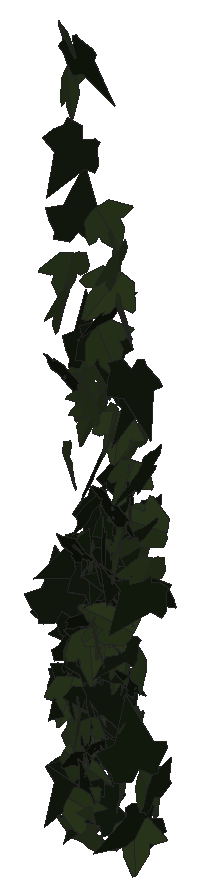
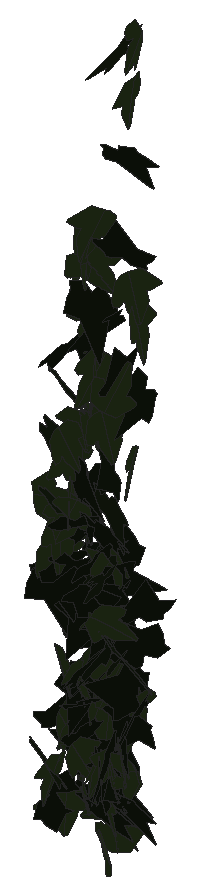
# SketchUp Ruby script. Lengths in inches.
U = 1.inch
M = Sketchup.active_model
def pt(a) = Geom::Point3d.new(a.map { |v| v * U })
def face(e, loops, mat)
  f = e.add_face(loops[0].map { |a| pt(a) })
  loops[1..].each { |l| e.add_face(l.map { |a| pt(a) }).erase! }
  f.material = f.back_material = mat if mat
  f
end
# faces: each face lists its corners as indices into pts; further lists are holes
def faces(e, pts, list, mat = nil) = list.each { |f| face(e, (f[0].is_a?(Array) ? f : [f]).map { |l| l.map { |i| pts[i] } }, mat) }
# xy, xz, yz: faces in a plane at the given z, y or x. An outline is a flat list of corners, or four numbers for a rectangle; further outlines are holes
def ring(l) = l.size == 4 ? [[l[0], l[1]], [l[2], l[1]], [l[2], l[3]], [l[0], l[3]]] : l.each_slice(2).to_a
def flat(e, list, mat, &to3) = list.each { |f| face(e, (f[0].is_a?(Array) ? f : [f]).map { |l| ring(l).map { |u, v| to3.(u, v) } }, mat) }
def xy(e, z, list, mat = nil) = flat(e, list, mat) { |x, y| [x, y, z] }
def xz(e, y, list, mat = nil) = flat(e, list, mat) { |x, z| [x, y, z] }
def yz(e, x, list, mat = nil) = flat(e, list, mat) { |y, z| [x, y, z] }
def lines(e, pts, list) = list.each { |a, b| e.add_line(pt(pts[a]), pt(pts[b])) }
# prism: a flat outline (further loops are holes) pulled along v
def prism(e, loops, v, mat = nil)
  f = face(e, loops, mat); d = Geom::Vector3d.new(v.map { |x| x * U })
  f.pushpull(f.normal.samedirection?(d) ? d.length : -d.length)
end
def box(e, o, s, mat = nil) = prism(e, [[o, [o[0] + s[0], o[1], o[2]], [o[0] + s[0], o[1] + s[1], o[2]], [o[0], o[1] + s[1], o[2]]]], [0, 0, s[2]], mat)
def at(x, y, z, deg = 0) = Geom::Transformation.translation(pt([x, y, z])) * Geom::Transformation.rotation(ORIGIN, Z_AXIS, deg.degrees)
def axes(o, x, y, z) = Geom::Transformation.new([*x, 0, *y, 0, *z, 0, *pt(o).to_a, 1])
def part(name) = M.definitions.add(name)
# library, detail: a bought-in or finely detailed component or shape, given as its bounding box
def library(name, o, s) = part(name).tap { |d| box(d.entities, o, s) }
def detail(e, o, s) = box(e.add_group.entities, o, s)
def put(e, d, t, mat = nil) = e.add_instance(d, t).tap { |i| i.material = mat if mat }
def group(e, t, mat = nil) = e.add_group.tap { |g| g.transformation = t; g.material = mat if mat }.entities
root = M.entities
M.materials.add("efeu1").color = [18, 25, 13]
M.materials.add("efeu2").color = [43, 57, 29]
c1 = part("ivyleaf_10")
p = [[0,0.5,-0.03],[-0.0625,2.02,-0.43],[-0.19,2.01,-0.46],[-0.54,1.05,-0.29],[-0.52,0.625,-0.18],[-0.83,0.76,-0.28],
  [-1.16,0.64,-0.33],[-1.15,0.33,-0.24],[-0.77,-0.39,0.02],[-0.3,-0.51,0.16],[0.04,-0.48,0.23],[-0.02,2.01,-0.4375],
  [-0.06,2.01,-0.43],[0.04,-0.49,0.23],[0.67,-0.49,0.14],[1.38,0.36,-0.2],[1.375,0.51,-0.24],[0.81,0.65,-0.19],
  [0.62,0.59,-0.15],[0.6,1.09,-0.28],[0.5,1.23,-0.31]]
faces(c1.entities,p,[[0,1,2,3,4,5,6,7,8,9,10],[11,12,0,13,14,15,16,17,18,19,20]],"efeu2")
c2 = part("ivyleaf_9")
p = [[1.54,2.16,1.25],[1.36,2.04,1.19],[-0.21,0.99,0.68],[-0.71,1.11,0.82],[-0.85,0.86,0.67],[-0.8,0.17,0.21],
  [-0.9,-0.01,0.1],[-0.67,-0.16,-0.02],[-0.08,-0.08,-0.05],[-0.03,-0.6,-0.4],[0.65,-0.88,-0.66],[0.83,-0.6,-0.49],
  [1.29,-0.42,-0.43],[1.8125,-0.07,-0.26],[1.21,0.44,0.15]]
faces(c2.entities,p,[[0,1,2,3,4,5,6,7,8,9,10,11,12,13,14]],"efeu1")
put(root,c1,axes([507.67,132.25,225.15],[-0.67169,0.30588,0.55125],[-0.57014,0.04902,-0.7219],[-0.26904,-0.86755,0.15357]))
put(root,c1,axes([506.41,132.4,240.61],[-0.63709,0.59964,-0.19778],[0.12594,-0.15195,-0.87449],[-0.66763,-0.60088,0.02377]))
put(root,c2,axes([506.32,132.27,215.31],[-0.63529,-0.37926,0.39302],[0.33878,0.21084,0.72786],[-0.46859,0.66662,-0.00661]))
put(root,c1,axes([507.2,132.45,210.73],[-0.86644,-0.09764,0.1844],[-0.173,-0.13686,-0.83213],[0.13365,-0.81014,0.11835]))
put(root,c1,axes([506.57,132.55,211.79],[0.53988,0.54531,-0.22704],[-0.16249,-0.15823,-0.76935],[-0.61321,0.52202,0.00397]))
put(root,c1,axes([507.625,132.41,214.31],[0.4981,0.73589,0.03065],[0.02054,0.02311,-0.8886],[-0.73624,0.49851,-0.00405]))
put(root,c1,axes([509.375,132.2,229.53],[-0.58306,0.57776,0.226],[-0.1394,0.17665,-0.82195],[-0.65192,-0.55451,-0.02637]))
put(root,c2,axes([507.05,133.03,207.83],[-0.06531,-0.25331,0.74015],[0.0799,-0.71251,-0.25721],[0.81193,0.04974,0.08485]))
put(root,c1,axes([508.6,132.67,230.33],[0.75093,0.29794,-0.48827],[-0.45735,-0.17118,-0.80784],[-0.34351,0.87921,0.00817]))
put(root,c1,axes([506.71,132.2,222.07],[-0.51143,0.56113,0.30999],[-0.22253,0.21604,-0.76342],[-0.64913,-0.51616,0.01748]))
put(root,c2,axes([506.87,132.48,240.15],[0.61355,-0.6211,-0.17687],[-0.01821,0.21235,-0.86517],[0.69524,0.55368,0.13342]))
put(root,c1,axes([508.78,132.77,218.96],[0.59224,-0.52273,0.26011],[0.21093,-0.15748,-0.78764],[0.58923,0.58177,0.02051]))
put(root,c1,axes([508.43,132.19,228.03],[0.27209,0.82406,0.33922],[-0.05181,0.3687,-0.85414],[-0.88964,0.23056,0.15349]))
put(root,c1,axes([508.94,132.8125,215.17],[0.25706,0.28657,0.81958],[-0.66136,-0.48916,0.37847],[0.56253,-0.70606,0.07044]))
put(root,c1,axes([507.16,132.65,205.33],[-0.85487,-0.08676,0.21494],[0.22177,0.02351,0.82814],[-0.09707,0.81775,-0.001]))
put(root,c1,axes([508.47,132.74,215.16],[0.51548,0.21436,-0.58934],[-0.59937,-0.13471,-0.53914],[-0.26249,0.72855,0.07371]))
put(root,c1,axes([507.45,132.5625,213.97],[0.71673,0.3637,0.15685],[0.1334,0.08834,-0.78682],[-0.40376,0.6748,0.01847]))
put(root,c2,axes([506.61,132.78,217.55],[0.43995,-0.34779,0.69724],[0.61992,-0.3525,-0.55291],[0.53014,0.70083,0.06791]))
put(root,c2,axes([506.74,132.97,235.77],[-0.83042,-0.30502,-0.14689],[0.15655,0.01725,-0.85943],[0.32753,-0.78158,0.03836]))
put(root,c1,axes([508.8,132.6,231.51],[0.12172,-0.9228,-0.18496],[-0.00907,0.18535,-0.93067],[0.94111,0.12114,0.01495]))
put(root,c1,axes([507.21,132.24,210.875],[0.2439,-0.41241,-0.64257],[-0.14472,0.61256,-0.47618],[0.78912,0.23981,0.11128]))
put(root,c2,axes([508.1,133.21,217.43],[0.04735,-0.60374,0.50972],[0.05813,-0.48736,-0.62936],[0.83783,0.06794,0.01486]))
put(root,c2,axes([508.39,132.27,218.23],[0.07473,-0.13769,0.80455],[-0.09498,0.77036,0.15078],[-0.84329,-0.09897,0.05432]))
put(root,c1,axes([507.07,132.41,206.8],[0.30052,0.18357,0.79237],[0.66513,0.44878,-0.34638],[-0.52343,0.67566,0.01479]))
put(root,c2,axes([509.31,132.94,226.49],[0.19125,-0.89939,-0.15714],[0.05764,0.17213,-0.915],[0.9112,0.17788,0.09086]))
put(root,c2,axes([509.89,132.56,209.49],[-0.8064,-0.36243,0.26858],[0.2402,0.12067,0.88403],[-0.38183,0.84134,-0.0111]))
put(root,c2,axes([507.9,132.96,227.62],[0.11037,-0.8961,-0.23053],[-0.02239,0.2295,-0.90286],[0.92501,0.11247,0.00565]))
put(root,c2,axes([509.76,133.375,206.68],[-0.17693,-0.13164,-0.83539],[0.18197,-0.83941,0.09373],[-0.82589,-0.15675,0.19962]))
put(root,c1,axes([507.4,133.07,224.46],[-0.01377,-0.86903,0.30995],[0.05038,-0.31023,-0.86757],[0.92127,0.00397,0.05208]))
put(root,c2,axes([507.08,133.14,213.09],[0.15733,-0.84779,0.09383],[0.01912,-0.09188,-0.86227],[0.85275,0.15848,0.00202]))
put(root,c1,axes([505.99,132.86,228.8],[0.22579,-0.90433,-0.06566],[-0.00115,0.06738,-0.93197],[0.90671,0.22528,0.01517]))
put(root,c2,axes([505.91,133.52,211.07],[-0.07322,-0.53236,0.72531],[-0.08075,-0.72088,-0.53726],[0.89608,-0.10846,0.01085]))
put(root,c1,axes([506.44,132.66,238.62],[-0.14614,0.84223,0.05058],[-0.15515,0.02554,-0.87554],[-0.89782,-0.1415,0.14306]))
put(root,c2,axes([508.68,132.47,220.64],[0.46788,0.25946,-0.72634],[-0.74399,-0.07221,-0.50504],[-0.2034,0.86097,0.17653]))
put(root,c2,axes([508.43,132.94,207.04],[-0.75249,0.1344,0.37809],[-0.38408,0.07571,-0.73795],[-0.16646,-0.78223,-0.00646]))
put(root,c1,axes([509.5,132.81,206.36],[0.61635,0.62959,0.01485],[0.00998,0.0109,-0.88374],[-0.68006,0.57077,0.00049]))
put(root,c1,axes([507.76,132.77,214.54],[-0.3113,0.70125,-0.07321],[0.03012,-0.06465,-0.78851],[-0.76056,-0.28958,-0.00125]))
put(root,c2,axes([508.01,132.8,212.14],[0.26587,-0.61638,-0.39674],[-0.06868,0.38296,-0.6862],[0.77985,0.24386,0.07482]))
put(root,c2,axes([507.7,132.22,221.15],[0.07249,0.32919,0.73978],[0.02554,0.71275,-0.34536],[-0.84612,0.04972,0.05295]))
put(root,c1,axes([506.18,133.02,230.26],[-0.36064,-0.74398,0.16557],[0.01049,-0.17801,-0.84399],[0.82162,-0.32429,0.08345]))
put(root,c2,axes([508,133.05,217.15],[0.47741,-0.62428,0.09278],[0.06374,-0.06751,-0.79548],[0.67809,0.44587,0.00945]))
put(root,c1,axes([507.04,132.96,217.97],[0.69693,-0.46021,-0.04305],[-0.03681,0.02349,-0.8243],[0.49767,0.64621,-0.00069]))
put(root,c1,axes([507.81,133.125,215.31],[0.17504,-0.70448,0.18481],[0.06667,-0.16806,-0.75145],[0.78183,0.17206,0.0227]))
put(root,c2,axes([507.64,132.53,219.96],[-0.3045,0.67694,0.28859],[-0.12358,0.25292,-0.7626],[-0.78042,-0.30417,0.00816]))
put(root,c1,axes([506.52,132.86,208.56],[-0.40923,-0.00883,-0.74078],[0.76754,-0.05982,-0.39241],[-0.05258,-0.80459,0.03731]))
put(root,c2,axes([509.64,133.55,216.98],[-0.53478,-0.66799,0.26634],[-0.11498,-0.24822,-0.85341],[0.70988,-0.54343,0.06242]))
put(root,c2,axes([507.3,132.41,215.34],[0.35075,0.67216,0.23948],[0.12811,0.19834,-0.7761],[-0.75658,0.34519,-0.02039]))
put(root,c1,axes([507.3,132.92,211.92],[-0.49395,0.60596,-0.05945],[-0.0404,0.04338,0.78954],[0.6561,0.45887,0.00386]))
put(root,c2,axes([506.9,133.52,213.33],[0.50755,-0.65826,-0.17136],[0.10526,-0.13287,0.84115],[-0.72526,-0.47995,0.00216]))
put(root,c2,axes([510.07,133.14,222.52],[-0.71206,0.44422,-0.27184],[0.16401,-0.23813,-0.81928],[-0.53194,-0.66807,0.11128]))
put(root,c1,axes([508.17,133.15,224],[0.59974,-0.56577,0.05282],[0.04239,-0.03263,-0.82445],[0.61202,0.55667,0.00535]))
put(root,c1,axes([507.9,133.26,214.95],[0.13032,0.61918,-0.42978],[-0.08366,-0.40592,-0.65606],[-0.7996,0.14339,-0.00141]))
put(root,c1,axes([508.66,133.0625,207.91],[0.51085,-0.61025,-0.13198],[-0.08845,0.09707,-0.80297],[0.66733,0.48002,-0.0054]))
put(root,c2,axes([508.625,133.31,214.375],[-0.792,-0.19176,-0.05415],[0.05325,0.01724,-0.7883],[0.20788,-0.73498,-0.00436]))
put(root,c2,axes([505.71,132.83,225.58],[0.84151,-0.03861,-0.23066],[-0.23925,0.01082,-0.81133],[0.0433,0.81005,-0.00016]))
put(root,c2,axes([507.32,132.66,209.17],[0.23771,0.78401,-0.0437],[-0.03192,-0.03534,-0.84667],[-0.84735,0.22128,0.01963]))
put(root,c2,axes([507.34,133.26,216.79],[-0.14376,-0.68839,-0.26187],[0.06814,0.24421,-0.72903],[0.7887,-0.14657,0.01525]))
put(root,c1,axes([507.2,133.04,210.87],[0.68311,0.40029,0.11152],[0.09533,0.06104,-0.77847],[-0.43729,0.63863,0.0045]))
put(root,c2,axes([506.3,133.36,207.59],[-0.86646,-0.11241,-0.22493],[0.23415,0.01091,-0.8423],[0.12031,-0.83085,0.01937]))
put(root,c2,axes([506.79,133.65,217.28],[-0.02705,-0.22374,-0.81976],[-0.10657,-0.78203,0.23412],[-0.87848,0.10176,-0.00317]))
put(root,c2,axes([507.4,133.33,206.94],[-0.85157,-0.07811,-0.1166],[0.11896,0.02519,-0.82391],[0.08733,-0.79602,-0.01463]))
put(root,c2,axes([507.06,132.5,207.78],[0.10923,0.31169,0.71141],[0.037,0.68759,-0.3311],[-0.81101,0.07335,0.08071]))
put(root,c1,axes([507.51,133.53,211.85],[-0.08398,0.38557,-0.65211],[-0.02793,-0.63156,-0.40055],[-0.79449,-0.01855,0.08301]))
put(root,c2,axes([507.29,133.1,208.08],[-0.24695,-0.07456,-0.79445],[-0.76978,-0.27506,0.2498],[-0.30751,0.74844,0.01266]))
put(root,c2,axes([507.51,133.7,217.88],[-0.17089,-0.84982,0.22084],[-0.0345,-0.21831,-0.86679],[0.87737,-0.17411,0.00893]))
put(root,c2,axes([506.98,132.88,210.84],[0.23506,-0.00332,-0.79278],[-0.82298,0.02032,-0.22636],[0.02209,0.79249,0.00248]))
put(root,c2,axes([508.17,133.52,214.3],[-0.72371,-0.26128,0.19819],[-0.17865,-0.09983,-0.74728],[0.30012,-0.68948,0.03309]))
put(root,c2,axes([507.19,132.82,211.81],[-0.02644,-0.22801,-0.74381],[0.07281,0.71203,-0.23848],[0.80745,-0.07167,-0.00285]))
put(root,c1,axes([509.21,132.78,220.14],[0.13305,-0.52193,-0.64525],[-0.16025,0.60244,-0.55771],[0.86084,0.19281,-0.00409]))
put(root,c1,axes([506.87,132.83,209.44],[-0.25401,0.30253,0.67506],[-0.61309,0.33773,-0.37763],[-0.47149,-0.60214,0.12735]))
put(root,c1,axes([507.15,133.13,209.0625],[0.4274,-0.62505,-0.28835],[-0.16051,0.23406,-0.76939],[0.72083,0.42273,-0.00035]))
put(root,c2,axes([508.25,132.83,228.9],[-0.14317,0.92607,-0.02665],[0.00489,-0.02621,-0.93707],[-0.92644,-0.14325,-0.00083]))
put(root,c1,axes([508.92,133.39,221.8],[0.35716,0.60352,-0.38465],[-0.25385,-0.29143,-0.71315],[-0.72108,0.40153,0.06054]))
put(root,c2,axes([509.19,133.74,216.49],[-0.28179,0.00115,0.84852],[-0.74388,-0.43046,-0.24646],[0.4082,-0.78365,0.13662]))
put(root,c1,axes([510.125,133.43,219.66],[0.07069,0.06033,0.90437],[-0.82332,-0.37508,0.08937],[0.37905,-0.82596,0.02547]))
put(root,c1,axes([508.3125,133.33,223.74],[0.83306,0.18053,0.01413],[0.01328,0.00709,-0.82388],[-0.19507,0.77144,0.00426]))
put(root,c2,axes([505.61,133.02,214.23],[-0.29276,-0.00659,0.79386],[0.82397,0.02465,0.282],[-0.02747,0.80966,-0.00212]))
put(root,c2,axes([509.05,133.72,225.22],[-0.711,-0.05027,-0.46968],[0.48232,-0.2183,-0.65179],[-0.09057,-0.76792,0.21603]))
put(root,c1,axes([507.9,133.15,226.04],[0.51447,-0.68339,-0.35174],[-0.01181,0.41618,-0.82588],[0.76851,0.46389,0.22277]))
put(root,c2,axes([507.37,133.66,219.49],[-0.78051,-0.1849,-0.40881],[0.40768,0.05031,-0.8011],[0.18737,-0.87965,0.04012]))
put(root,c2,axes([507.48,133.26,209.11],[0.24047,-0.14725,0.71263],[0.74384,-0.08716,-0.25223],[0.14016,0.71519,0.11598]))
put(root,c1,axes([509.52,133.62,217.67],[-0.26526,-0.82491,0.24159],[-0.01378,-0.24871,-0.86438],[0.85945,-0.25858,0.0607]))
put(root,c2,axes([505.85,133.5,211.53],[-0.44859,-0.25016,-0.65228],[0.58509,0.31608,-0.50424],[0.43531,-0.68264,0.00556]))
put(root,c1,axes([506.05,133.47,209.05],[-0.46488,0.09174,-0.67844],[0.66109,-0.23231,-0.45403],[-0.26296,-0.74624,0.05794]))
put(root,c1,axes([507.21,133.41,207.625],[0.61115,-0.48713,-0.21098],[-0.1603,0.13851,-0.77649],[0.54689,0.58497,0.00817]))
put(root,c1,axes([508.82,133.79,210.51],[0.20054,-0.75179,0.37403],[0.13078,-0.35189,-0.77741],[0.82945,0.23725,0.03214]))
put(root,c2,axes([509.78,133.56,220.03],[-0.71048,0.38665,-0.08026],[-0.00258,-0.15403,-0.78138],[-0.42581,-0.64421,0.13866]))
put(root,c2,axes([506.86,133.32,214.3125],[-0.62741,0.54168,0.27851],[-0.24866,0.1372,-0.82703],[-0.55601,-0.6726,0.05559]))
put(root,c1,axes([507.58,133.11,226.24],[-0.35576,-0.63603,-0.57077],[0.24752,0.51507,-0.72823],[0.81795,-0.4325,-0.02789]))
put(root,c1,axes([506.61,133.34,213.2],[-0.68759,-0.31143,-0.29301],[0.26255,0.14392,-0.73678],[0.36984,-0.68117,-0.02171]))
put(root,c2,axes([508.68,133.28,221.41],[-0.08758,0.01539,-0.90292],[-0.89994,-0.07679,0.08598],[-0.07496,0.9039,0.02268]))
put(root,c2,axes([508.03,133.97,210.3],[-0.23475,-0.70361,0.0718],[-0.02433,-0.0653,-0.76587],[0.76316,-0.21851,-0.00233]))
put(root,c2,axes([508.31,133.76,219.39],[-0.28416,-0.63698,-0.35202],[0.22937,0.27591,-0.7117],[0.74449,-0.32813,0.08491]))
put(root,c1,axes([506.83,133.625,217.86],[0.62445,0.0516,0.48969],[0.50689,0.03785,-0.6037],[-0.06903,0.7447,-0.00325]))
put(root,c1,axes([508.03,133.73,213.29],[0.1327,0.67237,-0.28158],[-0.04608,-0.26742,-0.71082],[-0.78146,0.12995,-0.0059]))
put(root,c2,axes([507.72,134.23,211.83],[-0.65811,-0.52279,0.2282],[0.0129,-0.36197,-0.79202],[0.57028,-0.59511,0.28127]))
put(root,c1,axes([507.59,133.22,232.64],[0.34933,0.66794,0.42368],[-0.00556,0.44264,-0.75052],[-0.84495,0.27324,0.1801]))
put(root,c1,axes([507.43,133.55,209.12],[-0.31145,0.66395,-0.05136],[0.02126,-0.0453,-0.75283],[-0.71874,-0.28905,-0.00001]))
put(root,c1,axes([506.45,134.02,225.4],[-0.42275,-0.51711,-0.48203],[-0.30383,-0.36835,0.67449],[-0.68567,0.48204,-0.00168]))
put(root,c2,axes([506.33,133.39,231.59],[-0.84074,0.05898,0.27968],[0.28989,-0.01688,0.81191],[0.06617,0.82343,-0.00339]))
put(root,c2,axes([507.875,133.24,215.57],[0.53231,0.57541,0.01798],[0.01234,0.01298,-0.78795],[-0.6216,0.49301,-0.00024]))
put(root,c1,axes([509.1,133.58,218.81],[-0.26052,-0.83736,-0.18676],[0.04519,0.18152,-0.87689],[0.85674,-0.2642,-0.01054]))
put(root,c2,axes([506.99,133.46,214.52],[0.70515,-0.19656,-0.32658],[-0.30872,0.13746,-0.70761],[0.2545,0.71134,0.04649]))
put(root,c2,axes([510.2,133.16,208],[-0.10996,0.52151,0.69024],[-0.38354,0.59429,-0.51011],[-0.77543,-0.3679,0.15443]))
put(root,c1,axes([507.55,134.16,231.07],[0.11154,-0.3213,0.75774],[0.58538,-0.50987,-0.31374],[0.63002,0.53062,0.15736]))
put(root,c1,axes([508.07,133.875,212.65],[0.65343,-0.40666,0.15366],[0.12678,-0.09018,-0.75809],[0.44975,0.61624,-0.00954]))
put(root,c1,axes([508.64,133.6,219.72],[-0.67946,-0.33795,-0.30661],[0.3152,0.07712,-0.73965],[0.36775,-0.69049,0.06746]))
put(root,c2,axes([506.86,133.25,209.93],[0.31393,-0.12072,-0.80522],[-0.65698,0.47222,-0.32693],[0.48096,0.72383,0.079]))
put(root,c2,axes([507.23,133.85,216.72],[-0.2786,-0.68816,-0.48894],[0.21288,0.44096,-0.74194],[0.81689,-0.34961,0.0266]))
put(root,c1,axes([509.16,133.65,213.1875],[0.54412,-0.48367,-0.34189],[-0.23064,0.25178,-0.72565],[0.58798,0.54636,0.03174]))
put(root,c1,axes([508.41,134.01,210.63],[-0.05429,0.56056,-0.46942],[-0.03134,-0.45368,-0.5826],[-0.77664,-0.02088,0.05632]))
put(root,c2,axes([508.01,133.47,212.46],[0.69192,0.2393,-0.33535],[-0.33714,-0.08509,-0.71071],[-0.27277,0.71217,0.02777]))
put(root,c2,axes([506.95,134.06,208.98],[0.01535,-0.06117,-0.76124],[0.7814,-0.12501,0.02548],[-0.13672,-0.72135,0.06014]))
put(root,c1,axes([509.53,133.46,208.24],[-0.13106,0.81365,0.25695],[-0.09794,0.2439,-0.82228],[-0.84761,-0.15399,0.05529]))
put(root,c1,axes([506.42,134.19,205.45],[0.01053,-0.15467,-0.77216],[0.44172,-0.62422,0.14083],[-0.68976,-0.40211,0.07839]))
put(root,c1,axes([508.65,134.06,223.11],[-0.12069,-0.71923,0.31529],[-0.02252,-0.3034,-0.75656],[0.84265,-0.11112,0.02494]))
put(root,c2,axes([506.5,133.49,226.05],[-0.24752,-0.45577,0.67241],[0.30761,0.58044,0.53054],[-0.79703,0.36556,-0.00406]))
put(root,c2,axes([507.96,134.16,212.75],[-0.06998,-0.87274,-0.00572],[-0.00874,-0.00504,0.8755],[-0.87272,0.07003,-0.00831]))
put(root,c2,axes([506.66,134.13,217.53],[0.34064,-0.60751,0.30609],[0.19262,-0.23832,-0.71038],[0.70315,0.3596,0.04632]))
put(root,c1,axes([506.85,134.03,215.7],[0.38367,0.18771,-0.64205],[-0.62821,-0.2119,-0.41512],[-0.30166,0.68002,0.04788]))
put(root,c1,axes([507.04,133.33,209.06],[0.01593,0.4524,0.61956],[-0.18127,0.58266,-0.45584],[-0.78728,-0.12501,0.11749]))
put(root,c2,axes([509.21,133.75,216.77],[0.42814,0.48634,-0.61673],[-0.3916,-0.47669,-0.64776],[-0.68083,0.58002,-0.01524]))
put(root,c1,axes([507.89,134.13,209.56],[-0.08324,-0.62584,0.3274],[-0.03318,-0.31338,-0.65575],[0.75587,-0.08268,0.00727]))
put(root,c1,axes([506.73,133.96,224.39],[-0.36406,-0.72312,0.1269],[-0.05926,-0.10904,-0.82973],[0.78979,-0.34151,-0.00376]))
put(root,c2,axes([505.81,133.33,212.49],[0.13814,0.07136,0.80918],[0.64881,0.49512,-0.14993],[-0.53953,0.61367,0.02688]))
